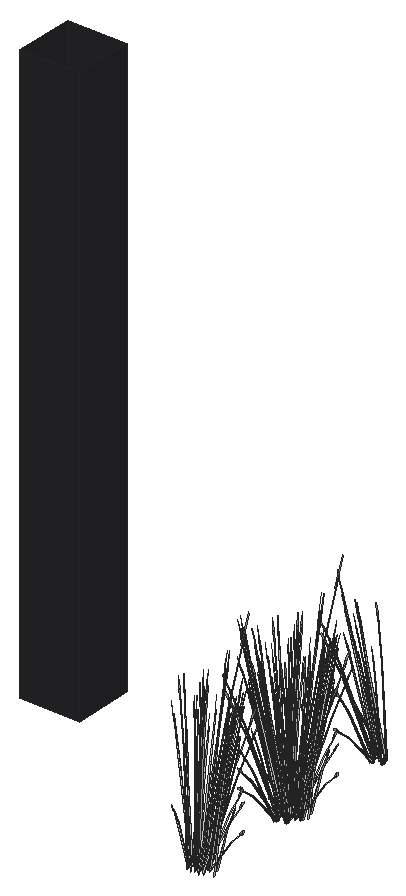
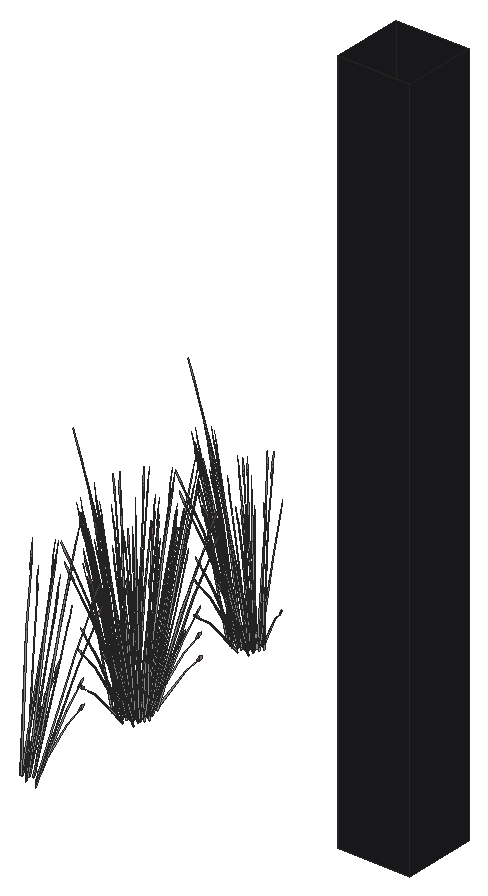
# SketchUp Ruby script. Lengths in inches.
U = 1.inch
M = Sketchup.active_model
def pt(a) = Geom::Point3d.new(a.map { |v| v * U })
def face(e, loops, mat)
  f = e.add_face(loops[0].map { |a| pt(a) })
  loops[1..].each { |l| e.add_face(l.map { |a| pt(a) }).erase! }
  f.material = f.back_material = mat if mat
  f
end
# faces: each face lists its corners as indices into pts; further lists are holes
def faces(e, pts, list, mat = nil) = list.each { |f| face(e, (f[0].is_a?(Array) ? f : [f]).map { |l| l.map { |i| pts[i] } }, mat) }
# xy, xz, yz: faces in a plane at the given z, y or x. An outline is a flat list of corners, or four numbers for a rectangle; further outlines are holes
def ring(l) = l.size == 4 ? [[l[0], l[1]], [l[2], l[1]], [l[2], l[3]], [l[0], l[3]]] : l.each_slice(2).to_a
def flat(e, list, mat, &to3) = list.each { |f| face(e, (f[0].is_a?(Array) ? f : [f]).map { |l| ring(l).map { |u, v| to3.(u, v) } }, mat) }
def xy(e, z, list, mat = nil) = flat(e, list, mat) { |x, y| [x, y, z] }
def xz(e, y, list, mat = nil) = flat(e, list, mat) { |x, z| [x, y, z] }
def yz(e, x, list, mat = nil) = flat(e, list, mat) { |y, z| [x, y, z] }
def lines(e, pts, list) = list.each { |a, b| e.add_line(pt(pts[a]), pt(pts[b])) }
# prism: a flat outline (further loops are holes) pulled along v
def prism(e, loops, v, mat = nil)
  f = face(e, loops, mat); d = Geom::Vector3d.new(v.map { |x| x * U })
  f.pushpull(f.normal.samedirection?(d) ? d.length : -d.length)
end
def box(e, o, s, mat = nil) = prism(e, [[o, [o[0] + s[0], o[1], o[2]], [o[0] + s[0], o[1] + s[1], o[2]], [o[0], o[1] + s[1], o[2]]]], [0, 0, s[2]], mat)
def at(x, y, z, deg = 0) = Geom::Transformation.translation(pt([x, y, z])) * Geom::Transformation.rotation(ORIGIN, Z_AXIS, deg.degrees)
def axes(o, x, y, z) = Geom::Transformation.new([*x, 0, *y, 0, *z, 0, *pt(o).to_a, 1])
def part(name) = M.definitions.add(name)
# library, detail: a bought-in or finely detailed component or shape, given as its bounding box
def library(name, o, s) = part(name).tap { |d| box(d.entities, o, s) }
def detail(e, o, s) = box(e.add_group.entities, o, s)
def put(e, d, t, mat = nil) = e.add_instance(d, t).tap { |i| i.material = mat if mat }
def group(e, t, mat = nil) = e.add_group.tap { |g| g.transformation = t; g.material = mat if mat }.entities
root = M.entities
M.materials.add("Asphalt_02_1K").color = [86, 76, 68]
M.materials.add("LightPink_Translucent").color = [144, 107, 117]
M.materials["LightPink_Translucent"].alpha = 0.75
M.materials.add("ThomThom - Buttons2").color = [40, 40, 43]
c1 = part("blade")
p = [[2.15,0.21,22],[0,0.17,0],[0.09,0.45,0],[2.18,0.31,22],[2.29,0.31,22],[0.38,0.45,0],
  [2.48,0.24,33],[2.49,0.24,33],[2.48,0.22,33]]
faces(c1.entities,p,[[0,1,2,3],[4,5,2,3],[6,3,4,7],[8,0,3,6]])
c2 = part("seeds")
p = [[0.3,-0.1,1.38],[-0.01,-0.03,1.59],[-0.01,-0.03,0.03],[0.14,-0.07,-0.07],[0.29,-0.03,3],[0.15,0.01,3.11]]
faces(c2.entities,p,[[0,1,2,3],[1,0,4,5]],"LightPink_Translucent")
c3 = part("blade with seeds")
put(c3.entities,c1,at(0,0,0))
put(c3.entities,c2,axes([2.4,0.25,30.99],[1.5799,-0.05474,1.17369],[-0.12525,1.92788,0.29478],[-0.07173,-0.02425,1.56792]))
xy(root,3,[[377,116.19,389,128.19]],"Asphalt_02_1K")
xz(root,116.19,[[377,3,389,120]],"ThomThom - Buttons2")
xz(root,128.19,[[377,3,389,120]],"ThomThom - Buttons2")
yz(root,377,[[116.19,3,128.19,120]],"ThomThom - Buttons2")
yz(root,389,[[116.19,3,128.19,120]],"ThomThom - Buttons2")
put(root,c3,axes([434.9,93.62,2.05],[-0.03403,-0.04831,1.5255],[0.07443,-0.51782,-0.14414],[0.13402,-0.03308,0.26996]))
put(root,c3,axes([430.47,91.52,2.05],[-0.06145,0.07164,1.50452],[0.00523,0.52344,-0.23794],[-0.14085,0.06807,0.12066]))
put(root,c3,axes([430.87,91.02,2.33],[0.18933,0.49965,-0.10458],[-0.33602,0.24554,-0.58045],[-0.1416,0.06592,0.88199]))
put(root,c3,axes([434.6,93.18,1.38],[-0.07202,-0.46385,-0.03003],[0.3404,-0.10664,-0.13615],[0.07108,0.02941,0.44908]))
put(root,c3,axes([433.72,93.17,2.33],[0.02015,-0.56117,-0.10458],[0.38148,0.01534,-0.58045],[0.14692,0.03898,0.88199]))
put(root,c3,axes([433.66,92.95,2.34],[-0.2141,-0.34548,0.30456],[0.24447,-0.32704,-0.39319],[0.12421,0.04976,0.75234]))
put(root,c3,axes([434.05,92.83,2.05],[0.08072,-0.00933,1.50452],[0.22141,-0.42869,-0.23794],[0.14358,0.05659,0.12066]))
put(root,c3,axes([430.82,92.41,2.07],[-0.09332,-0.50785,0.41282],[0.36608,-0.08814,0.34039],[-0.10789,0.11944,0.85423]))
put(root,c3,axes([430.75,92.32,2.07],[-0.25832,-0.23207,0.0553],[0.1504,-0.33047,0.43534],[-0.08282,0.10684,0.66383]))
put(root,c3,axes([430.87,91.7,1.33],[0.13056,-0.11672,1.47384],[0.10992,0.53933,0.11917],[-0.20497,0.12189,0.63005]))
put(root,c3,axes([431.05,92.25,2.34],[0.32754,-0.07886,0.30456],[0.08649,0.45081,-0.39319],[-0.09386,0.12109,0.75234]))
put(root,c3,axes([429.79,92.04,2.05],[0.04802,0.0148,1.5255],[0.14856,0.48754,-0.14414],[-0.0983,0.12796,0.26996]))
put(root,c3,axes([433.86,93.26,2.07],[-0.01895,0.4196,0.0553],[-0.28611,-0.0115,0.43534],[0.1096,0.04391,0.66383]))
put(root,c3,axes([433.88,93.13,2.07],[-0.27746,0.36359,0.41282],[-0.23929,-0.38612,0.34039],[0.13017,0.06707,0.85423]))
put(root,c3,axes([430.31,93.53,2.86],[0.33205,0.14729,-0.05579],[-0.10214,0.45334,-0.25298],[-0.05431,0.06883,0.83441]))
put(root,c3,axes([433,93.55,2.34],[-0.05812,-0.44446,0.30456],[0.33222,-0.11736,-0.39319],[0.08923,0.12737,0.75234]))
put(root,c3,axes([433.2,92.25,1.33],[-0.13977,-0.09507,1.47384],[0.28925,-0.39884,0.11917],[0.18028,0.17992,0.63005]))
put(root,c3,axes([433.22,90.99,1.85],[-0.32515,-0.2867,1.18923],[0.34333,-0.44639,0.51312],[0.10491,0.26901,1.1495]))
put(root,c3,axes([430.88,92.2,2.33],[0.34807,0.30426,-0.10458],[-0.20053,0.44063,-0.58045],[-0.09834,0.15317,0.88199]))
put(root,c3,axes([432.97,93.78,2.33],[0.22423,-0.47232,-0.10458],[0.32472,0.27211,-0.58045],[0.11288,0.13344,0.88199]))
put(root,c3,axes([431.35,92.07,1.33],[0.09398,-0.16955,1.47384],[0.23731,0.45764,0.11917],[-0.16276,0.20841,0.63005]))
put(root,c3,axes([431.49,93.14,2.34],[0.2546,-0.29052,0.30456],[0.24101,0.33173,-0.39319],[-0.03667,0.16855,0.75234]))
put(root,c3,axes([432.68,94.17,2.05],[0.00111,-0.06681,1.5255],[0.32247,-0.29474,-0.14414],[0.11201,0.1052,0.26996]))
put(root,c3,axes([431.26,93.41,2.07],[-0.30922,-0.02571,0.0553],[0.00848,-0.38824,0.43534],[-0.03236,0.14872,0.66383]))
put(root,c3,axes([431.36,93.44,2.07],[-0.26795,-0.37649,0.41282],[0.28456,-0.3247,0.34039],[-0.04943,0.17664,0.85423]))
put(root,c3,axes([432.21,93.62,2.34],[0.11344,-0.42434,0.30456],[0.33096,0.12377,-0.39319],[0.03035,0.17085,0.75234]))
put(root,c3,axes([433.05,93.95,2.07],[-0.17102,0.35053,0.0553],[-0.24354,-0.20408,0.43534],[0.07874,0.11238,0.66383]))
put(root,c3,axes([432.65,95.13,2.86],[0.26003,-0.31656,-0.05579],[0.23826,0.3467,-0.25298],[0.01677,0.09824,0.83441]))
put(root,c3,axes([433.125,93.86,2.07],[-0.37426,0.12663,0.41282],[-0.06495,-0.49674,0.34039],[0.08802,0.1464,0.85423]))
put(root,c3,axes([431.28,92.49,1.33],[0.07006,-0.18966,1.47384],[0.29392,0.3925,0.11917],[-0.13259,0.24463,0.63005]))
put(root,c3,axes([432.1,94.01,2.07],[-0.27727,0.18753,0.0553],[-0.13571,-0.34197,0.43534],[0.02678,0.15075,0.66383]))
put(root,c3,axes([430.48,93.47,2.05],[-0.00935,0.1092,1.50452],[0.26544,0.37987,-0.23794],[-0.06949,0.17964,0.12066]))
put(root,c3,axes([431.33,93.22,2.64],[0.41355,0.02734,-0.11608],[-0.0113,0.51765,-0.6443],[-0.02873,0.19937,0.97901]))
put(root,c3,axes([432.09,93.8,2.33],[0.36822,-0.25691,-0.10458],[0.18095,0.45596,-0.58045],[0.04858,0.19215,0.88199]))
put(root,c3,axes([432.2,93.97,2.35],[-0.37078,-0.14426,0.45823],[0.12679,-0.47426,0.37783],[0.02228,0.18651,0.9482]))
put(root,c3,axes([432.62,92.8,1.33],[-0.08601,-0.17716,1.47384],[0.39746,-0.14915,0.11917],[0.08983,0.27813,0.63005]))
put(root,c3,axes([430.45,94.59,2.05],[0.04269,-0.03331,1.5255],[0.35284,0.2216,-0.14414],[-0.00829,0.1845,0.26996]))
put(root,c3,axes([431.92,92.89,1.33],[-0.00921,-0.21179,1.47384],[0.39917,0.1405,0.11917],[-0.02469,0.30182,0.63005]))
put(root,c3,axes([432.01,94.82,2.05],[0.0477,0.08886,1.50452],[0.38493,0.03491,-0.23794],[0.03871,0.19596,0.12066]))
put(root,c3,axes([431.68,113.02,1.33],[0.08601,0.17716,1.47384],[-0.39746,0.14915,0.11917],[-0.08983,-0.27813,0.63005]))
put(root,c3,axes([432.33,111.84,2.05],[-0.05755,-0.07737,1.50452],[-0.38409,0.04905,-0.23794],[-0.0613,-0.18505,0.12066]))
put(root,c3,axes([434.06,112.79,2.05],[-0.00363,-0.10982,1.50452],[-0.30678,-0.3174,-0.23794],[0.04743,-0.1924,0.12066]))
put(root,c3,axes([433.02,113.33,1.33],[-0.07006,0.18966,1.47384],[-0.29392,-0.3925,0.11917],[0.13259,-0.24463,0.63005]))
put(root,c3,axes([433.98,112.4,2.05],[-0.03821,0.04215,1.5255],[-0.37441,-0.1422,-0.14414],[-0.01355,-0.18393,0.26996]))
put(root,c3,axes([431.9375,111.59,2.05],[-0.00702,0.06614,1.5255],[-0.34622,0.24004,-0.14414],[-0.10188,-0.1227,0.26996]))
put(root,c3,axes([431.86,112.76,2.38],[0.41917,-0.14183,0.46236],[0.07275,0.55635,0.38124],[-0.09858,-0.16397,0.95674]))
put(root,c3,axes([432.81,112.87,2.07],[0.37078,0.14426,0.41282],[-0.12679,0.47426,0.34039],[-0.02228,-0.18651,0.85423]))
put(root,c3,axes([432.92,113.04,2.33],[-0.36822,0.25691,-0.10458],[-0.18095,-0.45596,-0.58045],[-0.04858,-0.19215,0.88199]))
put(root,c3,axes([433.68,113.61,2.33],[-0.41355,-0.02734,-0.10458],[0.0113,-0.51765,-0.58045],[0.02873,-0.19937,0.88199]))
put(root,c3,axes([432.91,112.83,2.07],[0.27727,-0.18753,0.0553],[0.13571,0.34197,0.43534],[-0.02678,-0.15075,0.66383]))
put(root,c3,axes([431.96,112.88,2.07],[0.17102,-0.35053,0.0553],[0.24354,0.20408,0.43534],[-0.07874,-0.11238,0.66383]))
put(root,c3,axes([431.1,113.57,1.33],[0.13977,0.09507,1.47384],[-0.28925,0.39884,0.11917],[-0.18028,-0.17992,0.63005]))
put(root,c3,axes([432.81,113.22,2.34],[-0.11344,0.42434,0.30456],[-0.33096,-0.12377,-0.39319],[-0.03035,-0.17085,0.75234]))
put(root,c3,axes([433.65,113.4,2.07],[0.26795,0.37649,0.41282],[-0.28456,0.3247,0.34039],[0.04943,-0.17664,0.85423]))
put(root,c3,axes([432.04,112.85,2.67],[-0.25113,0.52899,-0.11713],[-0.36369,-0.30476,-0.65011],[-0.12642,-0.14945,0.98783]))
put(root,c3,axes([433.75,113.43,2.07],[0.30922,0.02571,0.0553],[-0.00848,0.38824,0.43534],[0.03236,-0.14872,0.66383]))
put(root,c3,axes([433.52,113.69,2.34],[-0.2546,0.29052,0.30456],[-0.24101,-0.33173,-0.39319],[0.03667,-0.16855,0.75234]))
put(root,c3,axes([431.07,112.7,2.05],[-0.08096,-0.00389,1.50452],[-0.25776,0.38949,-0.23794],[-0.13753,-0.07958,0.12066]))
put(root,c3,axes([434.13,114.63,2.33],[-0.34807,-0.30426,-0.10458],[0.20053,-0.44063,-0.58045],[0.09834,-0.15317,0.88199]))
put(root,c3,axes([432.01,113.29,2.34],[0.05812,0.44446,0.30456],[-0.33222,0.11736,-0.39319],[-0.08923,-0.12737,0.75234]))
put(root,c3,axes([431.01,113.58,2.38],[0.31075,-0.40722,0.46236],[0.268,0.43246,0.38124],[-0.14579,-0.07512,0.95674]))
put(root,c3,axes([434.99,114.5,2.05],[-0.04915,-0.00419,1.5255],[-0.20409,-0.44904,-0.14414],[0.08196,-0.14765,0.26996]))
put(root,c3,axes([431.16,113.57,2.07],[0.01895,-0.4196,0.0553],[0.28611,0.0115,0.43534],[-0.1096,-0.04391,0.66383]))
put(root,c3,axes([433.96,114.59,2.34],[-0.32754,0.07886,0.30456],[-0.08649,-0.45081,-0.39319],[0.09386,-0.12109,0.75234]))
put(root,c3,axes([434.26,114.52,2.07],[0.25832,0.23207,0.0553],[-0.1504,0.33047,0.43534],[0.08282,-0.10684,0.66383]))
put(root,c3,axes([434.1875,114.42,2.07],[0.09332,0.50785,0.41282],[-0.36608,0.08814,0.34039],[0.10789,-0.11944,0.85423]))
put(root,c3,axes([435.17,115.04,2.05],[0.05222,-0.08405,1.50452],[-0.06683,-0.51557,-0.23794],[0.13101,-0.09775,0.12066]))
put(root,c3,axes([430.76,113.03,2.05],[0.0279,0.05507,1.5255],[-0.13448,0.49501,-0.14414],[-0.1362,0.00358,0.26996]))
put(root,c3,axes([431.35,113.89,2.34],[0.2141,0.34548,0.30456],[-0.24447,0.32704,-0.39319],[-0.12421,-0.04976,0.75234]))
put(root,c3,axes([431.29,113.67,2.33],[-0.02015,0.56117,-0.10458],[-0.38148,-0.01534,-0.58045],[-0.14692,-0.03898,0.88199]))
put(root,c3,axes([434.15,115.82,2.33],[-0.18933,-0.49965,-0.10458],[0.33602,-0.24554,-0.58045],[0.1416,-0.06592,0.88199]))
put(root,c3,axes([430.81,114.44,1.33],[0.15608,-0.0125,1.47384],[-0.10354,0.54165,0.11917],[-0.22242,-0.0335,0.63005]))
put(root,c3,axes([434.01,115.67,2.34],[-0.31272,-0.15393,0.30456],[0.09121,-0.44909,-0.39319],[0.1259,-0.04118,0.75234]))
put(root,c3,axes([430.74,114.85,2.07],[0.10631,-0.50312,0.41282],[0.34951,0.17204,0.34039],[-0.13745,0.03024,0.85423]))
put(root,c3,axes([430.71,114.72,2.07],[-0.1382,-0.37624,0.0553],[0.25202,-0.18416,0.43534],[-0.11109,0.03633,0.66383]))
put(root,c3,axes([433.49,115.06,1.33],[-0.15608,0.0125,1.47384],[0.10354,-0.54165,0.11917],[0.22242,0.0335,0.63005]))
put(root,c3,axes([434.3,115.81,2.07],[0.1382,0.37624,0.0553],[-0.25202,0.18416,0.43534],[0.11109,-0.03633,0.66383]))
put(root,c3,axes([434.27,115.68,2.07],[-0.10631,0.50312,0.41282],[-0.34951,-0.17204,0.34039],[0.13745,-0.03024,0.85423]))
put(root,c3,axes([431,114.86,2.34],[0.31272,0.15393,0.30456],[-0.09121,0.44909,-0.39319],[-0.1259,0.04118,0.75234]))
put(root,c3,axes([434.9,117.31,2.05],[-0.03403,-0.04831,1.5255],[0.07443,-0.51782,-0.14414],[0.13402,-0.03308,0.26996]))
put(root,c3,axes([430.47,115.2,2.05],[-0.06145,0.07164,1.50452],[0.00523,0.52344,-0.23794],[-0.14085,0.06807,0.12066]))
put(root,c3,axes([430.87,114.71,2.33],[0.18933,0.49965,-0.10458],[-0.33602,0.24554,-0.58045],[-0.1416,0.06592,0.88199]))
put(root,c3,axes([434.6,116.87,1.38],[-0.07202,-0.46385,-0.03003],[0.3404,-0.10664,-0.13615],[0.07108,0.02941,0.44908]))
put(root,c3,axes([433.72,116.86,2.33],[0.02015,-0.56117,-0.10458],[0.38148,0.01534,-0.58045],[0.14692,0.03898,0.88199]))
put(root,c3,axes([433.66,116.64,2.34],[-0.2141,-0.34548,0.30456],[0.24447,-0.32704,-0.39319],[0.12421,0.04976,0.75234]))
put(root,c3,axes([434.05,116.52,2.05],[0.08072,-0.00933,1.50452],[0.22141,-0.42869,-0.23794],[0.14358,0.05659,0.12066]))
put(root,c3,axes([430.82,116.1,2.07],[-0.09332,-0.50785,0.41282],[0.36608,-0.08814,0.34039],[-0.10789,0.11944,0.85423]))
put(root,c3,axes([430.75,116.01,2.07],[-0.25832,-0.23207,0.0553],[0.1504,-0.33047,0.43534],[-0.08282,0.10684,0.66383]))
put(root,c3,axes([430.87,115.39,1.33],[0.13056,-0.11672,1.47384],[0.10992,0.53933,0.11917],[-0.20497,0.12189,0.63005]))
put(root,c3,axes([431.05,115.93,2.34],[0.32754,-0.07886,0.30456],[0.08649,0.45081,-0.39319],[-0.09386,0.12109,0.75234]))
put(root,c3,axes([429.79,115.73,2.05],[0.04802,0.0148,1.5255],[0.14856,0.48754,-0.14414],[-0.0983,0.12796,0.26996]))
put(root,c3,axes([433.86,116.95,2.07],[-0.01895,0.4196,0.0553],[-0.28611,-0.0115,0.43534],[0.1096,0.04391,0.66383]))
put(root,c3,axes([433.88,116.82,2.07],[-0.27746,0.36359,0.41282],[-0.23929,-0.38612,0.34039],[0.13017,0.06707,0.85423]))
put(root,c3,axes([430.31,117.21,2.86],[0.33205,0.14729,-0.05579],[-0.10214,0.45334,-0.25298],[-0.05431,0.06883,0.83441]))
put(root,c3,axes([433,117.24,2.34],[-0.05812,-0.44446,0.30456],[0.33222,-0.11736,-0.39319],[0.08923,0.12737,0.75234]))
put(root,c3,axes([433.2,115.93,1.33],[-0.13977,-0.09507,1.47384],[0.28925,-0.39884,0.11917],[0.18028,0.17992,0.63005]))
put(root,c3,axes([433.22,114.68,1.85],[-0.32515,-0.2867,1.18923],[0.34333,-0.44639,0.51312],[0.10491,0.26901,1.1495]))
put(root,c3,axes([430.88,115.89,2.33],[0.34807,0.30426,-0.10458],[-0.20053,0.44063,-0.58045],[-0.09834,0.15317,0.88199]))
put(root,c3,axes([432.97,117.47,2.33],[0.22423,-0.47232,-0.10458],[0.32472,0.27211,-0.58045],[0.11288,0.13344,0.88199]))
put(root,c3,axes([431.35,115.76,1.33],[0.09398,-0.16955,1.47384],[0.23731,0.45764,0.11917],[-0.16276,0.20841,0.63005]))
put(root,c3,axes([431.49,116.83,2.34],[0.2546,-0.29052,0.30456],[0.24101,0.33173,-0.39319],[-0.03667,0.16855,0.75234]))
put(root,c3,axes([432.68,117.86,2.05],[0.00111,-0.06681,1.5255],[0.32247,-0.29474,-0.14414],[0.11201,0.1052,0.26996]))
put(root,c3,axes([431.26,117.1,2.07],[-0.30922,-0.02571,0.0553],[0.00848,-0.38824,0.43534],[-0.03236,0.14872,0.66383]))
put(root,c3,axes([431.36,117.13,2.07],[-0.26795,-0.37649,0.41282],[0.28456,-0.3247,0.34039],[-0.04943,0.17664,0.85423]))
put(root,c3,axes([432.21,117.31,2.34],[0.11344,-0.42434,0.30456],[0.33096,0.12377,-0.39319],[0.03035,0.17085,0.75234]))
put(root,c3,axes([433.05,117.64,2.07],[-0.17102,0.35053,0.0553],[-0.24354,-0.20408,0.43534],[0.07874,0.11238,0.66383]))
put(root,c3,axes([432.65,118.82,2.86],[0.26003,-0.31656,-0.05579],[0.23826,0.3467,-0.25298],[0.01677,0.09824,0.83441]))
put(root,c3,axes([433.125,117.54,2.07],[-0.37426,0.12663,0.41282],[-0.06495,-0.49674,0.34039],[0.08802,0.1464,0.85423]))
put(root,c3,axes([431.28,116.17,1.33],[0.07006,-0.18966,1.47384],[0.29392,0.3925,0.11917],[-0.13259,0.24463,0.63005]))
put(root,c3,axes([432.1,117.69,2.07],[-0.27727,0.18753,0.0553],[-0.13571,-0.34197,0.43534],[0.02678,0.15075,0.66383]))
put(root,c3,axes([430.48,117.16,2.05],[-0.00935,0.1092,1.50452],[0.26544,0.37987,-0.23794],[-0.06949,0.17964,0.12066]))
put(root,c3,axes([431.33,116.91,2.64],[0.41355,0.02734,-0.11608],[-0.0113,0.51765,-0.6443],[-0.02873,0.19937,0.97901]))
put(root,c3,axes([432.09,117.49,2.33],[0.36822,-0.25691,-0.10458],[0.18095,0.45596,-0.58045],[0.04858,0.19215,0.88199]))
put(root,c3,axes([432.2,117.66,2.35],[-0.37078,-0.14426,0.45823],[0.12679,-0.47426,0.37783],[0.02228,0.18651,0.9482]))
put(root,c3,axes([432.62,116.49,1.33],[-0.08601,-0.17716,1.47384],[0.39746,-0.14915,0.11917],[0.08983,0.27813,0.63005]))
put(root,c3,axes([430.45,118.28,2.05],[0.04269,-0.03331,1.5255],[0.35284,0.2216,-0.14414],[-0.00829,0.1845,0.26996]))
put(root,c3,axes([431.92,116.57,1.33],[-0.00921,-0.21179,1.47384],[0.39917,0.1405,0.11917],[-0.02469,0.30182,0.63005]))
put(root,c3,axes([432.01,118.51,2.05],[0.0477,0.08886,1.50452],[0.38493,0.03491,-0.23794],[0.03871,0.19596,0.12066]))
put(root,c3,axes([431.68,137.13,1.33],[0.08601,0.17716,1.47384],[-0.39746,0.14915,0.11917],[-0.08983,-0.27813,0.63005]))
put(root,c3,axes([432.33,135.95,2.05],[-0.05755,-0.07737,1.50452],[-0.38409,0.04905,-0.23794],[-0.0613,-0.18505,0.12066]))
put(root,c3,axes([434.06,136.9,2.05],[-0.00363,-0.10982,1.50452],[-0.30678,-0.3174,-0.23794],[0.04743,-0.1924,0.12066]))
put(root,c3,axes([433.02,137.44,1.33],[-0.07006,0.18966,1.47384],[-0.29392,-0.3925,0.11917],[0.13259,-0.24463,0.63005]))
put(root,c3,axes([433.98,136.51,2.05],[-0.03821,0.04215,1.5255],[-0.37441,-0.1422,-0.14414],[-0.01355,-0.18393,0.26996]))
put(root,c3,axes([431.9375,135.7,2.05],[-0.00702,0.06614,1.5255],[-0.34622,0.24004,-0.14414],[-0.10188,-0.1227,0.26996]))
put(root,c3,axes([431.86,136.875,2.38],[0.41917,-0.14183,0.46236],[0.07275,0.55635,0.38124],[-0.09858,-0.16397,0.95674]))
put(root,c3,axes([432.81,136.98,2.07],[0.37078,0.14426,0.41282],[-0.12679,0.47426,0.34039],[-0.02228,-0.18651,0.85423]))
put(root,c3,axes([432.92,137.15,2.33],[-0.36822,0.25691,-0.10458],[-0.18095,-0.45596,-0.58045],[-0.04858,-0.19215,0.88199]))
put(root,c3,axes([433.68,137.73,2.33],[-0.41355,-0.02734,-0.10458],[0.0113,-0.51765,-0.58045],[0.02873,-0.19937,0.88199]))
put(root,c3,axes([432.91,136.94,2.07],[0.27727,-0.18753,0.0553],[0.13571,0.34197,0.43534],[-0.02678,-0.15075,0.66383]))
put(root,c3,axes([431.96,136.99,2.07],[0.17102,-0.35053,0.0553],[0.24354,0.20408,0.43534],[-0.07874,-0.11238,0.66383]))
put(root,c3,axes([431.1,137.68,1.33],[0.13977,0.09507,1.47384],[-0.28925,0.39884,0.11917],[-0.18028,-0.17992,0.63005]))
put(root,c3,axes([432.81,137.33,2.34],[-0.11344,0.42434,0.30456],[-0.33096,-0.12377,-0.39319],[-0.03035,-0.17085,0.75234]))
put(root,c3,axes([433.65,137.51,2.07],[0.26795,0.37649,0.41282],[-0.28456,0.3247,0.34039],[0.04943,-0.17664,0.85423]))
